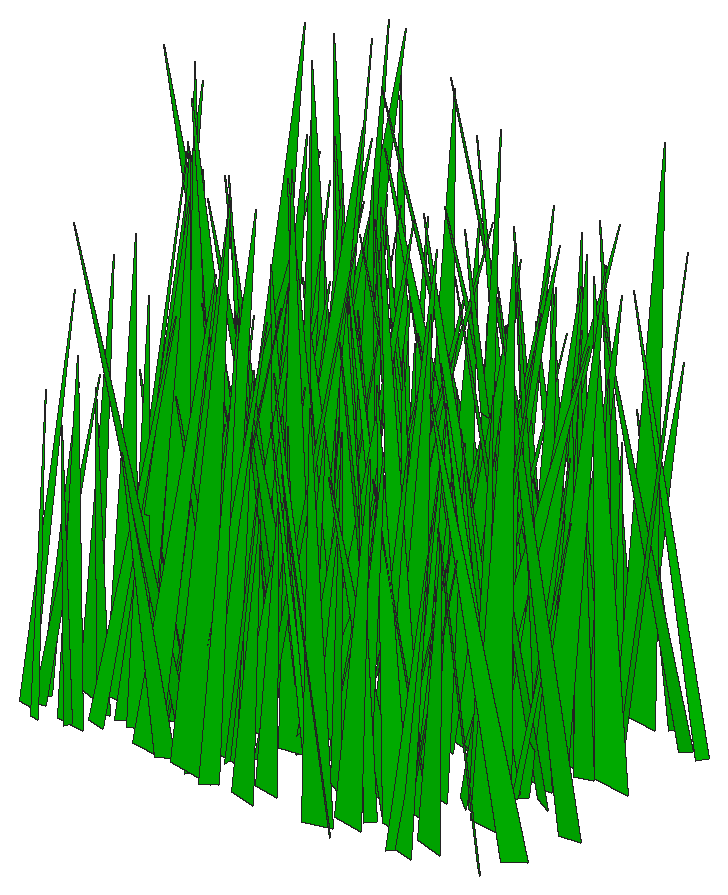
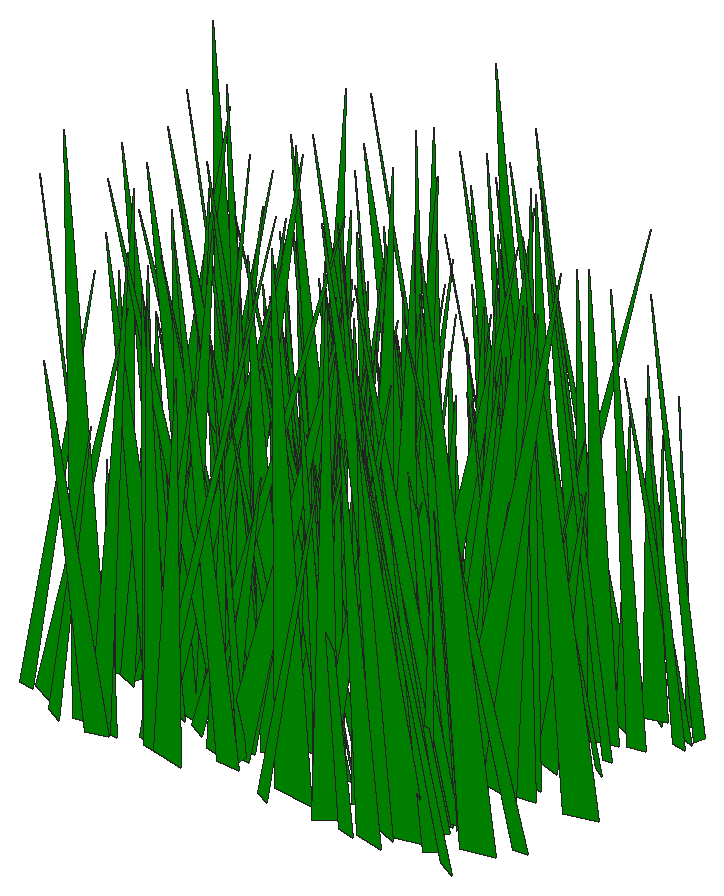
# SketchUp Ruby script. Lengths in inches.
U = 1.inch
M = Sketchup.active_model
def pt(a) = Geom::Point3d.new(a.map { |v| v * U })
def face(e, loops, mat)
  f = e.add_face(loops[0].map { |a| pt(a) })
  loops[1..].each { |l| e.add_face(l.map { |a| pt(a) }).erase! }
  f.material = f.back_material = mat if mat
  f
end
# faces: each face lists its corners as indices into pts; further lists are holes
def faces(e, pts, list, mat = nil) = list.each { |f| face(e, (f[0].is_a?(Array) ? f : [f]).map { |l| l.map { |i| pts[i] } }, mat) }
# xy, xz, yz: faces in a plane at the given z, y or x. An outline is a flat list of corners, or four numbers for a rectangle; further outlines are holes
def ring(l) = l.size == 4 ? [[l[0], l[1]], [l[2], l[1]], [l[2], l[3]], [l[0], l[3]]] : l.each_slice(2).to_a
def flat(e, list, mat, &to3) = list.each { |f| face(e, (f[0].is_a?(Array) ? f : [f]).map { |l| ring(l).map { |u, v| to3.(u, v) } }, mat) }
def xy(e, z, list, mat = nil) = flat(e, list, mat) { |x, y| [x, y, z] }
def xz(e, y, list, mat = nil) = flat(e, list, mat) { |x, z| [x, y, z] }
def yz(e, x, list, mat = nil) = flat(e, list, mat) { |y, z| [x, y, z] }
def lines(e, pts, list) = list.each { |a, b| e.add_line(pt(pts[a]), pt(pts[b])) }
# prism: a flat outline (further loops are holes) pulled along v
def prism(e, loops, v, mat = nil)
  f = face(e, loops, mat); d = Geom::Vector3d.new(v.map { |x| x * U })
  f.pushpull(f.normal.samedirection?(d) ? d.length : -d.length)
end
def box(e, o, s, mat = nil) = prism(e, [[o, [o[0] + s[0], o[1], o[2]], [o[0] + s[0], o[1] + s[1], o[2]], [o[0], o[1] + s[1], o[2]]]], [0, 0, s[2]], mat)
def at(x, y, z, deg = 0) = Geom::Transformation.translation(pt([x, y, z])) * Geom::Transformation.rotation(ORIGIN, Z_AXIS, deg.degrees)
def axes(o, x, y, z) = Geom::Transformation.new([*x, 0, *y, 0, *z, 0, *pt(o).to_a, 1])
def part(name) = M.definitions.add(name)
# library, detail: a bought-in or finely detailed component or shape, given as its bounding box
def library(name, o, s) = part(name).tap { |d| box(d.entities, o, s) }
def detail(e, o, s) = box(e.add_group.entities, o, s)
def put(e, d, t, mat = nil) = e.add_instance(d, t).tap { |i| i.material = mat if mat }
def group(e, t, mat = nil) = e.add_group.tap { |g| g.transformation = t; g.material = mat if mat }.entities
root = M.entities
M.materials.add("[Color G06]").color = [0, 204, 0]
c1 = part("fur_instance\#9")
p = [[0.8125,0,1.79],[0.67,-0.02,1.48],[0,-0.11,0],[0,0.11,0]]
faces(c1.entities,p,[[0,1,2,3]])
put(root,c1,axes([91.95,21.32,4.28],[1.64465,0.73134,2.25033],[5.45141,-0.21076,-1.03131],[0.23572,-0.22861,8.1499]),"[Color G06]")
put(root,c1,axes([92.71,15.9,4.28],[2.99438,-0.06344,1.89199],[-0.62767,-0.4469,0.49765],[-1.18975,0.07611,4.49924]),"[Color G06]")
put(root,c1,axes([92.1,16.31,4.28],[4.0526,-0.14556,1.75837],[-1.22143,-0.57694,0.80167],[-0.99093,0.11582,6.20302]),"[Color G06]")
put(root,c1,axes([92.28,16.91,4.28],[3.05677,-0.19884,0.87659],[-1.37312,-0.43367,-0.60473],[-0.70131,-0.01757,5.0048]),"[Color G06]")
put(root,c1,axes([92.375,16.52,4.28],[2.99104,0.29547,0.37118],[2.10052,-0.4183,0.44185],[-0.37328,0.01376,5.46057]),"[Color G06]")
put(root,c1,axes([94.8,22.62,4.28],[2.21877,0.53293,5.82163],[4.74581,-0.47788,0.9851],[-2.69366,-0.40297,6.5309]),"[Color G06]")
put(root,c1,axes([93.6,16.14,4.28],[2.27486,0.22768,1.51712],[1.48655,-0.34736,1.00952],[-1.21924,0.00129,4.06149]),"[Color G06]")
put(root,c1,axes([93.07,17.67,4.28],[3.03492,0.39872,2.50768],[3.18932,-0.43774,-0.62669],[-0.9051,-0.2055,6.20035]),"[Color G06]")
put(root,c1,axes([93.63,16.2,4.28],[-1.08085,0.50633,0.55689],[3.62015,0.15563,-0.55976],[0.46648,-0.03458,5.6344]),"[Color G06]")
put(root,c1,axes([94.27,19.8125,4.28],[-0.50605,0.37921,1.58428],[2.87616,0.03927,0.97251],[-0.49659,-0.15902,4.01814]),"[Color G06]")
put(root,c1,axes([92.85,24.4,4.28],[1.81921,0.75767,2.15229],[5.62004,-0.24113,-0.85976],[0.10756,-0.21572,8.52053]),"[Color G06]")
put(root,c1,axes([94.36,21.62,4.28],[1.43029,-0.58528,3.25632],[-4.53769,-0.25922,-0.90006],[-1.33139,0.25473,6.56581]),"[Color G06]")
put(root,c1,axes([93.08,19.76,4.28],[1.51262,0.3388,0.84647],[2.49354,-0.20247,-0.64393],[0.07692,-0.09865,4.22869]),"[Color G06]")
put(root,c1,axes([92.03,23.69,4.28],[4.42501,0.36233,0.30572],[2.60635,-0.61553,-0.46422],[-0.01867,-0.0518,7.65535]),"[Color G06]")
put(root,c1,axes([94,17.08,4.28],[2.06067,0.31223,1.61538],[2.21047,-0.31969,0.79948],[-1.13822,-0.05557,4.47718]),"[Color G06]")
put(root,c1,axes([93.82,21.51,4.28],[-0.60566,-0.69279,0.93666],[-4.99182,0.0905,0.47974],[0.3968,0.08111,7.4649]),"[Color G06]")
put(root,c1,axes([93.07,19.2,4.28],[2.93871,0.17543,0.30847],[1.22542,-0.40864,0.6195],[-0.3516,0.04202,4.73731]),"[Color G06]")
put(root,c1,axes([94.08,20.89,4.28],[4.11121,-0.516,3.26399],[-3.85509,-0.6291,-0.57814],[-1.89747,0.16013,8.24663]),"[Color G06]")
put(root,c1,axes([93.92,17.93,4.28],[-1.43333,0.57089,2.63425],[4.36949,0.23095,-0.43888],[0.88024,-0.21683,6.46806]),"[Color G06]")
put(root,c1,axes([92.95,25.57,4.28],[3.76983,0.29249,0.11472],[2.07066,-0.52185,0.85143],[-0.34352,0.06427,6.39126]),"[Color G06]")
put(root,c1,axes([95.07,22.84,4.28],[-2.9575,-0.53591,0.43812],[-3.81178,0.41431,0.74025],[0.57108,-0.00997,7.20988]),"[Color G06]")
put(root,c1,axes([93.25,18.61,4.28],[5.58813,-0.10913,1.7411],[-0.71926,-0.79537,-0.57038],[-1.2051,-0.03134,8.41406]),"[Color G06]")
put(root,c1,axes([94.03,23.76,4.28],[2.93262,0.05641,1.41875],[0.59159,-0.41868,-0.81912],[-0.84545,-0.09728,4.34804]),"[Color G06]")
put(root,c1,axes([93.76,25.09,4.28],[1.35656,-0.37728,0.80661],[-2.75127,-0.17878,0.72969],[0.20459,0.09739,4.46423]),"[Color G06]")
put(root,c1,axes([94.75,24.08,4.28],[-1.97383,0.26013,0.5172],[1.76197,0.27715,-0.99228],[0.70359,0.03569,3.93588]),"[Color G06]")
put(root,c1,axes([94.69,18.97,4.28],[1.16364,-0.67512,3.34217],[-5.32923,-0.15917,0.45111],[-0.19991,0.31342,7.42835]),"[Color G06]")
put(root,c1,axes([94.53,23.07,4.28],[-0.46455,0.6645,2.60656],[4.99984,0.10165,-0.98646],[0.86674,-0.23023,7.08753]),"[Color G06]")
put(root,c1,axes([94.46,21.07,4.28],[3.42196,-0.19032,0.99506],[-1.30572,-0.48562,-0.63985],[-0.77539,-0.02219,5.46887]),"[Color G06]")
put(root,c1,axes([94.74,22.9,4.28],[0.39123,-0.56087,0.88439],[-4.04925,-0.04637,0.62342],[0.36261,0.08738,6.00752]),"[Color G06]")
put(root,c1,axes([95.92,20.8,4.28],[-1.70962,0.30842,0.79986],[2.27481,0.23405,0.49352],[0.059,-0.0873,4.14878]),"[Color G06]")
put(root,c1,axes([95.11,17.1,4.28],[3.13375,-0.39209,1.95253],[-2.87491,-0.46445,-0.40724],[-1.16087,0.0918,6.27937]),"[Color G06]")
put(root,c1,axes([94.47,23.73,4.28],[4.2554,-0.27939,1.23783],[-1.95141,-0.60445,-0.68723],[-0.94461,-0.00994,6.99603]),"[Color G06]")
put(root,c1,axes([96.55,19.83,4.28],[-2.49548,0.77239,0.426],[5.54426,0.34621,0.43851],[-0.15085,-0.05302,9.06921]),"[Color G06]")
put(root,c1,axes([94.13,16.61,4.28],[4.2348,-0.19544,1.12768],[-1.51164,-0.58747,0.98408],[-0.49864,0.1211,6.59383]),"[Color G06]")
put(root,c1,axes([97.25,16.5625,4.28],[-4.59793,-0.36372,0.46774],[-2.6267,0.63798,-0.68693],[0.044,0.0773,7.87078]),"[Color G06]")
put(root,c1,axes([94.18,24.25,4.28],[3.85342,-0.32238,0.85745],[-2.37548,-0.53133,0.89846],[-0.17576,0.11325,6.65582]),"[Color G06]")
put(root,c1,axes([96.08,20.73,4.28],[-4.52783,0.15917,2.66712],[1.40693,0.66496,0.77652],[1.58369,-0.13566,6.93557]),"[Color G06]")
put(root,c1,axes([95.37,25.71,4.28],[1.86018,0.53518,0.62372],[3.82813,-0.26406,0.52574],[-0.49945,-0.03069,6.35262]),"[Color G06]")
put(root,c1,axes([95.9,22.22,4.28],[0.58753,-0.52227,1.63752],[-3.86787,-0.09841,-0.50568],[-0.51706,0.14272,5.64348]),"[Color G06]")
put(root,c1,axes([95.6875,19.57,4.28],[-2.50721,-0.37686,1.81547],[-2.6715,0.38349,0.90351],[1.28157,0.06213,5.43509]),"[Color G06]")
put(root,c1,axes([94.43,23.67,4.28],[3.53534,0.5577,0.76514],[4.03176,-0.4901,-0.57566],[-0.04827,-0.08908,7.95719]),"[Color G06]")
put(root,c1,axes([94.59,25.02,4.28],[2.2635,0.80743,1.04085],[5.81948,-0.30588,-1.01146],[0.3822,-0.12448,9.23651]),"[Color G06]")
put(root,c1,axes([96.15,23.26,4.28],[-1.78077,0.31236,0.47134],[2.21083,0.25217,-0.53936],[0.47889,-0.00264,4.24274]),"[Color G06]")
put(root,c1,axes([96.32,23.34,4.28],[0.37297,0.80273,1.56889],[5.81494,-0.06722,0.86282],[-0.65308,-0.14005,8.57838]),"[Color G06]")
put(root,c1,axes([94.71,17.29,4.28],[4.34523,-0.58439,0.34625],[-4.14669,-0.60491,-1.04009],[-0.6491,-0.04762,8.96239]),"[Color G06]")
put(root,c1,axes([95.05,21.3,4.28],[2.09902,0.42207,1.37893],[3.16426,-0.27995,-0.91564],[0.00054,-0.15444,5.42838]),"[Color G06]")
put(root,c1,axes([96.59,16.34,4.28],[-0.45543,-0.40546,0.95129],[-2.93274,0.04578,-0.89476],[-0.5087,0.09907,4.30676]),"[Color G06]")
put(root,c1,axes([96.84,17.41,4.28],[-2.89233,-0.0914,0.36995],[-0.61413,0.40129,0.6644],[0.33727,-0.05312,4.38233]),"[Color G06]")
put(root,c1,axes([95.33,25.125,4.28],[4.87842,0.45836,2.23764],[3.29222,-0.7086,0.64133],[-1.48574,-0.06514,8.76839]),"[Color G06]")
put(root,c1,axes([95.68,18.75,4.28],[-1.11238,0.64458,2.21192],[4.75124,0.18787,-0.95173],[0.99156,-0.17708,7.04181]),"[Color G06]")
put(root,c1,axes([97.89,19.89,4.28],[-4.06494,-0.02811,0.27236],[-0.22865,0.5597,-0.98594],[0.14689,0.09321,6.00238]),"[Color G06]")
put(root,c1,axes([95.63,17.9375,4.28],[4.09226,0.49238,1.39853],[3.51284,-0.58419,0.66672],[-1.00181,-0.03715,8.05069]),"[Color G06]")
put(root,c1,axes([95.69,23.86,4.28],[5.90719,-0.15838,2.43731],[-1.02526,-0.85381,-0.82302],[-1.70244,-0.03537,8.9527]),"[Color G06]")
put(root,c1,axes([96.12,25.7,4.28],[3.19355,-0.23482,0.85311],[-1.60083,-0.45093,-0.87237],[-0.7739,-0.03625,5.32493]),"[Color G06]")
put(root,c1,axes([96.95,25.49,4.28],[3.54346,-0.40804,4.40308],[-3.76669,-0.54316,0.98885],[-1.74751,0.34336,6.79678]),"[Color G06]")
put(root,c1,axes([97.75,17.88,4.28],[-1.76497,-0.43414,0.22457],[-3.10942,0.24356,-0.49855],[-0.21666,0.04111,5.32554]),"[Color G06]")
put(root,c1,axes([97.13,23.24,4.28],[3.75132,-0.61056,3.41678],[-4.53662,-0.58422,-0.86668],[-1.95359,0.18427,8.57359]),"[Color G06]")
put(root,c1,axes([96.54,24.28,4.28],[-0.44673,-0.68146,0.96305],[-4.88803,0.07288,0.85925],[0.6357,0.0815,7.28378]),"[Color G06]")
put(root,c1,axes([96.03,21.27,4.28],[1.87379,0.52475,1.07318],[3.82757,-0.25173,-0.78863],[0.16166,-0.1222,6.2332]),"[Color G06]")
put(root,c1,axes([98.05,24.19,4.28],[-3.83242,0.27082,1.38135],[2.08696,0.53192,0.95406],[0.52013,-0.13883,6.35003]),"[Color G06]")
put(root,c1,axes([98.47,19.72,4.28],[-3.59612,-0.54162,0.50753],[-3.89888,0.49945,-0.48125],[-0.00648,0.06525,7.89645]),"[Color G06]")
put(root,c1,axes([96.56,18.17,4.28],[0.81207,0.75992,0.72789],[5.46522,-0.10943,-0.49565],[0.25764,-0.07389,8.21978]),"[Color G06]")
put(root,c1,axes([97.32,19.21,4.28],[0.75766,-0.55761,1.57953],[-4.10077,-0.12081,-0.50553],[-0.53941,0.13522,6.06178]),"[Color G06]")
put(root,c1,axes([95.97,16.37,4.28],[3.6282,-0.49221,1.51641],[-3.65759,-0.50226,0.82028],[-0.33262,0.15402,7.52081]),"[Color G06]")
put(root,c1,axes([96.2,16.72,4.28],[3.48639,0.09583,0.67061],[0.6484,-0.489,0.49755],[-0.50318,0.03386,5.28758]),"[Color G06]")
put(root,c1,axes([96.81,22.35,4.28],[4.00358,0.04241,1.86246],[0.46894,-0.57849,-0.73852],[-1.19394,-0.085,5.95526]),"[Color G06]")
put(root,c1,axes([97.37,21.48,4.28],[1.89763,0.56922,1.9269],[4.20339,-0.28499,0.42443],[-0.81028,-0.14534,6.71448]),"[Color G06]")
put(root,c1,axes([96.2,23.37,4.28],[4.81694,-0.0289,1.13678],[-0.14184,-0.67775,-0.63675],[-0.77547,-0.05555,7.17774]),"[Color G06]")
put(root,c1,axes([98.3,19.2,4.28],[-3.66356,-0.29535,0.89766],[-2.03706,0.51643,0.94899],[0.83507,-0.03598,6.25309]),"[Color G06]")
put(root,c1,axes([96.22,17.97,4.28],[4.6601,0.03494,0.83555],[0.21637,-0.65342,0.44321],[-0.57316,0.03741,6.96082]),"[Color G06]")
put(root,c1,axes([96.91,21.89,4.28],[3.11215,-0.62531,0.6525],[-4.46156,-0.43803,-0.68761],[-0.62721,0.01314,8.1289]),"[Color G06]")
put(root,c1,axes([97.22,25.13,4.28],[3.51474,-0.2617,2.18796],[-2.10302,-0.51195,0.51204],[-1.11467,0.14069,5.93293]),"[Color G06]")
put(root,c1,axes([97.04,19.875,4.28],[1.73365,0.35845,0.83397],[2.63005,-0.23779,-0.47171],[-0.04451,-0.08918,4.60991]),"[Color G06]")
put(root,c1,axes([98.89,21.6,4.28],[-2.5379,0.1495,0.36355],[1.09806,0.34882,0.64508],[0.0527,-0.06869,4.06677]),"[Color G06]")
put(root,c1,axes([98.94,25.59,4.28],[-3.18182,-0.21847,0.9028],[-1.63005,0.44521,-0.45629],[0.40309,0.07582,5.28104]),"[Color G06]")
put(root,c1,axes([98.05,20,4.28],[-4.68369,-0.32627,4.29429],[-2.96612,0.71717,-0.96689],[2.22088,0.26974,7.76503]),"[Color G06]")
put(root,c1,axes([97.18,20.6,4.28],[1.74898,0.83775,0.49469],[6.00903,-0.24076,-0.61942],[0.30617,-0.06039,9.33119]),"[Color G06]")
put(root,c1,axes([97.7,17.31,4.28],[1.02984,0.50211,1.90448],[3.81912,-0.13247,-0.60111],[0.06009,-0.18614,5.56502]),"[Color G06]")
put(root,c1,axes([98.57,21.72,4.28],[-4.09565,0.42448,3.12993],[3.39886,0.60381,0.52775],[1.44907,-0.2165,7.60854]),"[Color G06]")
put(root,c1,axes([97.36,18.84,4.28],[2.99256,-0.29017,1.13786],[-2.18836,-0.41504,0.6975],[-0.34773,0.11469,5.4028]),"[Color G06]")
put(root,c1,axes([98.5,22.02,4.28],[2.51636,-0.19004,1.81097],[-1.24024,-0.38944,-0.84508],[-1.33689,0.00359,4.19271]),"[Color G06]")
put(root,c1,axes([97.61,16.125,4.28],[0.02228,0.70307,4.68772],[5.88419,0.05605,-1.0282],[0.79646,-0.43377,7.46505]),"[Color G06]")
put(root,c1,axes([98.76,20.03,4.28],[0.93266,-0.7566,1.56566],[-5.45628,-0.14954,-1.0409],[-0.87475,0.12606,8.16201]),"[Color G06]")
put(root,c1,axes([97.98,17.15,4.28],[2.66516,0.17119,0.78651],[1.10653,-0.37471,0.99352],[-0.7481,0.05563,4.27153]),"[Color G06]")
put(root,c1,axes([98.39,23.27,4.28],[-1.41919,-0.41651,0.91922],[-2.96636,0.21049,0.726],[0.70736,0.04706,4.88877]),"[Color G06]")
put(root,c1,axes([98.33,25.08,4.28],[1.4761,0.76761,1.12378],[5.53414,-0.21272,0.45425],[-0.49057,-0.09006,8.50575]),"[Color G06]")
put(root,c1,axes([98.63,24.75,4.28],[-2.2068,-0.21807,1.04001],[-1.48492,0.32265,0.73349],[0.85133,-0.00248,3.97529]),"[Color G06]")
put(root,c1,axes([98.43,23.78,4.28],[-1.98118,0.35268,1.1502],[2.45384,0.29522,-0.9575],[0.98365,-0.02614,4.70525]),"[Color G06]")
put(root,c1,axes([99.125,20.22,4.28],[-0.49134,0.44469,1.22671],[3.26056,0.04951,0.8554],[-0.46067,-0.12387,4.74598]),"[Color G06]")
put(root,c1,axes([97.53,22.77,4.28],[3.13387,-0.13497,0.45801],[-0.99727,-0.43524,0.50819],[-0.19044,0.05804,4.87571]),"[Color G06]")
put(root,c1,axes([100.03,23.51,4.28],[-4.35536,0.09656,0.82743],[0.77067,0.60368,0.9682],[0.43831,-0.1019,6.51967]),"[Color G06]")
put(root,c1,axes([98.85,18.72,4.28],[2.64629,0.14895,2.4302],[1.51659,-0.39771,-0.88866],[-1.21857,-0.1715,4.17154]),"[Color G06]")
put(root,c1,axes([99.66,20.125,4.28],[-2.03847,0.52015,1.88665],[3.93797,0.26896,0.98599],[-0.00588,-0.19861,6.27618]),"[Color G06]")
put(root,c1,axes([98.48,19.53,4.28],[0.36446,-0.40217,1.47164],[-3.03445,-0.0351,0.57672],[0.28184,0.14214,4.30626]),"[Color G06]")
put(root,c1,axes([99.07,18.62,4.28],[1.48161,0.74655,2.37301],[5.51387,-0.23181,0.68769],[-0.88324,-0.19485,8.2737]),"[Color G06]")
put(root,c1,axes([98.32,15.97,4.28],[4.13606,-0.3473,1.80889],[-2.47609,-0.59967,-0.57962],[-1.23974,0.03902,7.19257]),"[Color G06]")
put(root,c1,axes([97.64,16.25,4.28],[4.59531,-0.3301,0.53237],[-2.31211,-0.63988,-0.99706],[-0.62024,-0.06034,7.66113]),"[Color G06]")
put(root,c1,axes([100.81,24.33,4.28],[-4.02186,0.48193,0.19408],[3.4508,0.55735,0.75217],[-0.23005,-0.06499,7.88962]),"[Color G06]")
put(root,c1,axes([99.45,21.88,4.28],[-3.73003,-0.00036,1.79175],[0.16936,0.5407,0.80006],[1.18681,-0.07829,5.5171]),"[Color G06]")
put(root,c1,axes([99.62,22.98,4.28],[2.61455,-0.40861,3.55022],[-3.28205,-0.44508,-0.48555],[-1.85935,0.21106,5.84927]),"[Color G06]")
put(root,c1,axes([98.16,22.95,4.28],[3.23565,0.08858,0.60938],[0.5611,-0.44966,0.85353],[-0.5049,0.06795,4.85376]),"[Color G06]")
put(root,c1,axes([99.49,22.45,4.28],[-3.71818,-0.37291,1.92629],[-2.69894,0.5446,0.47446],[1.23637,0.06736,6.82872]),"[Color G06]")
put(root,c1,axes([97.97,23.67,4.28],[1.89484,0.51387,0.57617],[3.68226,-0.25445,-0.98062],[0.41196,-0.08922,6.11499]),"[Color G06]")
put(root,c1,axes([99,19.77,4.28],[-0.57469,0.3872,0.37092],[2.7551,0.08428,-0.57125],[0.42555,-0.02274,4.19926]),"[Color G06]")
put(root,c1,axes([100.21,21.28,4.28],[-4.43487,0.16092,1.93047],[1.35698,0.63048,0.92616],[1.07641,-0.13183,6.78605]),"[Color G06]")
put(root,c1,axes([100.85,23.9,4.28],[-2.41203,0.35942,0.31934],[2.58193,0.33225,0.60489],[-0.15102,-0.06024,5.24117]),"[Color G06]")
put(root,c1,axes([99.44,15.93,4.28],[-0.04825,-0.45111,0.02317],[-3.19754,0.00698,0.73431],[0.4915,0.00111,4.77949]),"[Color G06]")
put(root,c1,axes([99.27,18.65,4.28],[0.5699,-0.38393,0.39747],[-2.72636,-0.07157,0.79025],[0.46714,0.05068,4.12722]),"[Color G06]")
put(root,c1,axes([100.57,17.3,4.28],[-3.40365,0.08463,1.41087],[0.7378,0.4855,0.6303],[0.84565,-0.08295,5.12866]),"[Color G06]")
put(root,c1,axes([99.7,16.58,4.28],[-0.06059,-0.41869,0.65791],[-3.01651,0.01501,0.47687],[0.33124,0.06012,4.46304]),"[Color G06]")
put(root,c1,axes([102.41,23.92,4.28],[-5.77783,-0.30153,0.16469],[-2.16513,0.8043,-0.50729],[-0.01595,0.04971,9.20639]),"[Color G06]")
put(root,c1,axes([98.01,22.7,4.28],[5.07071,0.26378,0.34059],[1.90523,-0.70285,-0.82848],[-0.01847,-0.08354,8.04618]),"[Color G06]")
put(root,c1,axes([98.4375,17.84,4.28],[5.68966,-0.09614,1.04279],[-0.63784,-0.7977,-0.67405],[-0.74516,-0.05123,8.53925]),"[Color G06]")
put(root,c1,axes([99.22,22.34,4.28],[2.67202,-0.39584,1.06861],[-2.92715,-0.36291,0.90634],[-0.03516,0.13064,5.7556]),"[Color G06]")
put(root,c1,axes([98.77,20.2,4.28],[5.19698,-0.32427,0.83159],[-2.30121,-0.72872,-0.51864],[-0.64934,-0.01275,8.49357]),"[Color G06]")
put(root,c1,axes([101.33,16.78,4.28],[-3.64074,0.32921,0.44436],[2.29786,0.5061,-1.01836],[0.61795,0.05763,6.40479]),"[Color G06]")
put(root,c1,axes([99.32,23.61,4.28],[2.94786,-0.20381,0.5567],[-1.50581,-0.4042,0.81238],[-0.08614,0.0911,4.85001]),"[Color G06]")
put(root,c1,axes([100.05,23.6,4.28],[0.28779,-0.65932,1.85026],[-4.86294,-0.02131,0.81741],[0.48953,0.17595,7.03227]),"[Color G06]")
put(root,c1,axes([101.29,24.16,4.28],[-1.05253,0.37713,0.91239],[2.76369,0.13546,0.68983],[-0.22096,-0.10217,4.28213]),"[Color G06]")
put(root,c1,axes([100.15,18.91,4.28],[1.94771,-0.2804,1.44269],[-2.22261,-0.259,0.91998],[-0.18747,0.15749,4.0816]),"[Color G06]")
put(root,c1,axes([100.24,18.77,4.28],[0.36675,0.37985,0.72745],[2.70978,-0.03543,-0.92629],[0.56051,-0.07724,4.00216]),"[Color G06]")
put(root,c1,axes([102.9,25.11,4.28],[-5.77934,-0.24182,0.81091],[-1.77438,0.80543,-0.65632],[0.39158,0.08058,8.99421]),"[Color G06]")
put(root,c1,axes([100.57,22.44,4.28],[-1.03723,-0.36571,1.48549],[-2.66824,0.17419,0.76471],[0.86396,0.09892,4.14515]),"[Color G06]")
put(root,c1,axes([100.57,24.39,4.28],[3.80207,-0.07969,1.92762],[-0.73628,-0.55311,0.61739],[-1.20328,0.08666,5.71303]),"[Color G06]")
put(root,c1,axes([101.68,18.77,4.28],[-3.99591,-0.15864,1.60701],[-1.10565,0.57702,0.40224],[1.10808,0.00368,6.19646]),"[Color G06]")
put(root,c1,axes([101.83,20.95,4.28],[-3.437,0.28494,1.87877],[2.29424,0.47993,1.01368],[0.70153,-0.1735,5.88954]),"[Color G06]")
put(root,c1,axes([101.02,22.2,4.28],[2.44796,0.29452,1.38655],[2.08762,-0.36309,0.62702],[-0.9816,-0.03771,4.79139]),"[Color G06]")
put(root,c1,axes([101.01,17.77,4.28],[-2.78855,-0.25123,2.11196],[-1.80018,0.43244,0.59986],[1.41493,0.05506,4.92546]),"[Color G06]")
put(root,c1,axes([101.28,24.54,4.28],[1.60422,-0.36688,0.90151],[-2.58975,-0.23678,-0.7755],[-0.76096,0.03241,4.53975]),"[Color G06]")
put(root,c1,axes([100.27,22.03,4.28],[2.11814,-0.35676,0.27225],[-2.55065,-0.28951,0.74614],[0.27028,0.06381,4.9078]),"[Color G06]")
put(root,c1,axes([101.78,19.29,4.28],[1.43867,0.36329,1.01685],[2.52108,-0.21952,1.0419],[-0.94574,-0.03254,4.32425]),"[Color G06]")
put(root,c1,axes([102.26,15.9375,4.28],[-3.42771,-0.09529,1.00947],[-0.55558,0.48127,1.0049],[0.7839,-0.07558,5.12621]),"[Color G06]")
put(root,c1,axes([101.65,19.92,4.28],[2.77164,-0.40639,1.85195],[-2.89668,-0.41814,-0.85672],[-1.27985,0.06629,5.94959]),"[Color G06]")
put(root,c1,axes([100.65,24.84,4.28],[4.30318,-0.39722,1.03958],[-2.81675,-0.60784,-0.63548],[-0.81486,0.00347,7.68665]),"[Color G06]")
put(root,c1,axes([101.32,18.4,4.28],[3.74901,-0.01047,1.87537],[0.07835,-0.54738,-0.70107],[-1.25459,-0.06548,5.56027]),"[Color G06]")
put(root,c1,axes([102.08,25.54,4.28],[0.53987,0.57931,0.50841],[4.12625,-0.08105,0.82162],[-0.5904,-0.03672,6.20708]),"[Color G06]")
put(root,c1,axes([100.95,22.8125,4.28],[4.09954,-0.01951,1.35761],[0.01119,-0.57792,-1.02949],[-0.919,-0.09406,6.04358]),"[Color G06]")
put(root,c1,axes([101.78,16.05,4.28],[1.05403,-0.62649,0.08558],[-4.47618,-0.14713,-0.57738],[-0.38917,-0.00456,6.87278]),"[Color G06]")
put(root,c1,axes([103.81,23.48,4.28],[-4.35322,-0.40246,0.37628],[-2.89573,0.60251,-0.8041],[-0.08892,0.0819,7.76472]),"[Color G06]")
put(root,c1,axes([101.89,22.47,4.28],[-1.70723,0.49139,1.98205],[3.66449,0.2635,-0.45379],[0.86496,-0.14643,5.83465]),"[Color G06]")
put(root,c1,axes([101.62,19.09,4.28],[2.71976,0.7023,0.27363],[5.00242,-0.37973,0.892],[-0.61193,0.01722,8.50805]),"[Color G06]")
put(root,c1,axes([103.14,17.41,4.28],[-1.15604,-0.45466,0.41842],[-3.22955,0.15182,-0.98011],[-0.52824,0.06679,5.0765]),"[Color G06]")
put(root,c1,axes([101.66,19.68,4.28],[3.04674,0.22109,0.81038],[1.50149,-0.42987,0.86232],[-0.74379,0.03785,5.06028]),"[Color G06]")
put(root,c1,axes([102.78,18.44,4.28],[3.26634,-0.476,5.08849],[-4.34222,-0.53964,0.42711],[-2.095,0.37635,7.04825]),"[Color G06]")
put(root,c1,axes([103.09,23.03,4.28],[-5.34813,0.2136,2.41468],[1.67015,0.77255,0.41223],[1.47218,-0.10046,8.30436]),"[Color G06]")
put(root,c1,axes([102.86,25.1875,4.28],[-0.5015,-0.50341,1.2561],[-3.68334,0.05445,-0.77818],[-0.4148,0.12514,5.39148]),"[Color G06]")
put(root,c1,axes([103.16,23.4375,4.28],[-0.78154,-0.48769,0.04301],[-3.4473,0.10672,-0.9132],[-0.59014,0.02244,5.27751]),"[Color G06]")
put(root,c1,axes([101.96,22.15,4.28],[-4.08873,-0.50227,4.1822],[-3.90084,0.65664,0.54028],[2.36372,0.21484,8.12594]),"[Color G06]")
put(root,c1,axes([101.89,18.1875,4.28],[2.1114,0.38285,1.62936],[2.93418,-0.29344,-0.57263],[-0.34211,-0.15391,5.14472]),"[Color G06]")
put(root,c1,axes([101.84,19.04,4.28],[4.08903,-0.12303,1.94108],[-1.08281,-0.58683,0.82238],[-1.13698,0.1164,6.19767]),"[Color G06]")
put(root,c1,axes([102.04,17.32,4.28],[1.01411,-0.4756,1.58302],[-3.57039,-0.13149,0.57111],[0.08203,0.1566,5.28728]),"[Color G06]")
put(root,c1,axes([103.29,22.4,4.28],[-3.89679,-0.48029,1.0827],[-3.39477,0.55268,0.87128],[0.92917,0.00498,7.72394]),"[Color G06]")
put(root,c1,axes([102.5,25.44,4.28],[2.04432,0.55439,1.69919],[4.04715,-0.30453,0.53746],[-0.8482,-0.11687,6.65987]),"[Color G06]")
put(root,c1,axes([102.74,16.99,4.28],[-2.79719,0.19062,2.18267],[1.66088,0.41643,0.57682],[1.11481,-0.14213,4.61721]),"[Color G06]")
put(root,c1,axes([102.36,16.56,4.28],[0.37862,-0.51111,1.44085],[-3.7774,-0.03991,0.59089],[0.30801,0.1388,5.47538]),"[Color G06]")
put(root,c1,axes([101.66,21.25,4.28],[3.69536,0.49897,1.55488],[3.71418,-0.50973,-0.92713],[-0.30167,-0.16358,7.63179]),"[Color G06]")
put(root,c1,axes([103.35,23.39,4.28],[-2.73951,-0.6019,1.21268],[-4.31567,0.39367,0.66814],[0.81529,0.06134,7.61154]),"[Color G06]")
put(root,c1,axes([104.42,20.32,4.28],[-3.57748,0.60307,0.89745],[4.36611,0.49501,0.66591],[0.03625,-0.10414,8.36208]),"[Color G06]")
put(root,c1,axes([103.51,17.07,4.28],[-2.61642,0.52014,0.36544],[3.68497,0.36588,-0.8909],[0.62791,0.02013,6.75107]),"[Color G06]")
put(root,c1,axes([102.54,18.73,4.28],[0.5412,-0.66744,1.87095],[-4.93882,-0.06254,0.62837],[0.29154,0.1796,7.17177]),"[Color G06]")
put(root,c1,axes([102.96,24.82,4.28],[-1.56615,0.59799,1.21148],[4.28001,0.23393,-0.90515],[0.85338,-0.07581,6.76296]),"[Color G06]")
put(root,c1,axes([101.54,22.55,4.28],[4.38792,0.15689,0.56469],[1.16554,-0.60769,-0.8353],[-0.2239,-0.08874,6.7185]),"[Color G06]")
put(root,c1,axes([102.12,21.51,4.28],[1.7097,0.71847,0.20895],[5.12057,-0.23442,-0.99472],[0.5882,-0.0476,8.05223]),"[Color G06]")
put(root,c1,axes([102.84,18.63,4.28],[3.7427,-0.12735,1.92339],[-1.10087,-0.54165,0.66524],[-1.13061,0.10583,5.7193]),"[Color G06]")
put(root,c1,axes([101.49,23.7,4.28],[4.36131,0.49254,0.25031],[3.53412,-0.6059,-0.58933],[0.11845,-0.05741,8.36714]),"[Color G06]")
put(root,c1,axes([104.39,17.47,4.28],[-3.42038,-0.04589,0.72051],[-0.28354,0.47993,0.50477],[0.51021,-0.04093,5.11074]),"[Color G06]")
put(root,c1,axes([101.73,21.9,4.28],[3.60302,-0.62278,0.47575],[-4.46608,-0.49583,0.99157],[0.31862,0.09249,8.51876]),"[Color G06]")
put(root,c1,axes([103.25,21.58,4.28],[-1.09257,0.39978,1.44473],[2.9182,0.17708,-0.69943],[0.7987,-0.10012,4.53181]),"[Color G06]")
put(root,c1,axes([103.17,19.05,4.28],[0.22653,0.49833,1.15609],[3.63894,-0.02017,-0.59393],[0.35711,-0.11057,5.31876]),"[Color G06]")
put(root,c1,axes([103.34,23.54,4.28],[3.168,0.36659,1.12223],[2.54523,-0.45396,0.98535],[-0.99833,0.00591,6.07331]),"[Color G06]")
put(root,c1,axes([102.83,17.72,4.28],[2.95295,0.0388,0.43446],[0.32722,-0.40627,-0.80005],[-0.2342,-0.07841,4.36016]),"[Color G06]")
put(root,c1,axes([104.32,20.17,4.28],[-2.92689,-0.29194,0.96436],[-2.04946,0.41793,0.63984],[0.77411,0.00265,5.34018]),"[Color G06]")
put(root,c1,axes([104.3,25.5,4.28],[-3.37021,-0.46933,1.79073],[-3.39005,0.4926,0.57909],[1.12731,0.07825,7.09503]),"[Color G06]")
put(root,c1,axes([104.02,25.4375,4.28],[2.04001,-0.22654,1.20551],[-1.62507,-0.30346,-0.40806],[-0.80553,0.03851,3.87617]),"[Color G06]")
put(root,c1,axes([103.68,17.94,4.28],[1.96291,-0.35689,2.21218],[-2.93098,-0.2674,0.85363],[-0.3879,0.21452,4.74443]),"[Color G06]")
put(root,c1,axes([103.77,22.34,4.28],[-0.02185,0.60026,2.88863],[4.70047,0.02638,-0.55018],[0.41329,-0.26824,6.41008]),"[Color G06]")
put(root,c1,axes([105.24,22.79,4.28],[-2.809,0.10085,0.09434],[0.71061,0.38916,-0.52651],[0.14853,0.04541,4.30309]),"[Color G06]")
put(root,c1,axes([105.6,20.43,4.28],[-4.78377,-0.28171,0.86283],[-1.9861,0.67162,0.59322],[0.68564,-0.02007,7.73842]),"[Color G06]")
put(root,c1,axes([102.625,21.4,4.28],[3.32425,0.49147,0.13692],[3.49907,-0.45775,-1.01584],[0.4323,-0.07424,7.16938]),"[Color G06]")
put(root,c1,axes([105.51,18.81,4.28],[-3.75314,0.37365,0.36468],[2.65034,0.52347,-0.68382],[0.46383,0.03233,6.85822]),"[Color G06]")
put(root,c1,axes([104.06,21.99,4.28],[0.1667,0.38235,0.07779],[2.71889,-0.02209,-0.5416],[0.35864,-0.01025,4.06972]),"[Color G06]")
put(root,c1,axes([103.61,23.89,4.28],[2.7635,-0.52121,1.18425],[-3.81742,-0.3824,0.56463],[-0.16135,0.12032,6.92443]),"[Color G06]")
put(root,c1,axes([105.16,21.03,4.28],[3.48557,0.34154,3.42547],[2.63882,-0.56374,0.45907],[-2.07091,-0.14348,6.35043]),"[Color G06]")
put(root,c1,axes([104.09,16.2,4.28],[2.81319,-0.21429,0.71109],[-1.50875,-0.39783,-0.43938],[-0.55827,-0.0047,4.77076]),"[Color G06]")
put(root,c1,axes([103.98,16.8125,4.28],[3.05215,0.0598,0.65281],[0.32701,-0.42113,1.01656],[-0.51746,0.0866,4.49291]),"[Color G06]")
put(root,c1,axes([104.54,22.47,4.28],[-0.11407,-0.50068,1.27791],[-3.67429,0.0267,0.46918],[0.34957,0.11729,5.3484]),"[Color G06]")
put(root,c1,axes([104.45,16.1875,4.28],[1.41507,0.30532,1.33696],[2.3534,-0.19627,-0.41512],[-0.23616,-0.12639,3.87419]),"[Color G06]")
put(root,c1,axes([104.08,21.3,4.28],[1.4709,0.71338,0.36206],[5.11503,-0.20284,-0.50663],[0.25931,-0.04547,7.93965]),"[Color G06]")
put(root,c1,axes([104.6875,18.94,4.28],[2.82887,0.36781,2.72273],[3.05713,-0.41147,-0.70966],[-0.9644,-0.22546,5.73699]),"[Color G06]")
put(root,c1,axes([105.43,22.99,4.28],[-2.23803,-0.26922,1.83562],[-2.21381,0.31535,-0.71609],[0.57876,0.16517,4.35911]),"[Color G06]")
put(root,c1,axes([104.29,25.64,4.28],[1.07645,0.50442,0.60655],[3.62342,-0.14286,-0.71605],[0.34703,-0.07297,5.59499]),"[Color G06]")
put(root,c1,axes([104.73,16.89,4.28],[-0.7318,-0.4648,0.31439],[-3.2633,0.1059,1.01827],[0.71092,0.00766,4.9977]),"[Color G06]")
put(root,c1,axes([104.73,25.28,4.28],[0.95098,0.7524,3.03853],[5.76579,-0.12187,-0.56428],[0.04455,-0.28828,8.16903]),"[Color G06]")
put(root,c1,axes([105.79,25.52,4.28],[-2.4432,-0.23163,1.36916],[-1.85207,0.33631,-0.84647],[0.41014,0.13887,4.33366]),"[Color G06]")
put(root,c1,axes([103.96,19.24,4.28],[5.13002,0.15036,1.57403],[1.22613,-0.71929,-1.03326],[-0.87659,-0.12617,7.76629]),"[Color G06]")
put(root,c1,axes([106.7,24.84,4.28],[-3.63629,-0.33093,0.87855],[-2.44237,0.49838,-1.01548],[0.11147,0.12431,6.40979]),"[Color G06]")
put(root,c1,axes([106.87,17.67,4.28],[-2.66838,0.52542,0.24649],[3.74459,0.36572,0.99658],[-0.45019,-0.07234,6.82826]),"[Color G06]")
put(root,c1,axes([105.57,22.13,4.28],[2.15341,0.4481,1.96646],[3.28288,-0.33307,0.68839],[-1.13139,-0.11356,5.74025]),"[Color G06]")
put(root,c1,axes([104.86,21.69,4.28],[2.72323,0.67036,0.46217],[4.79322,-0.38201,0.56334],[-0.48054,-0.01148,8.23836]),"[Color G06]")
put(root,c1,axes([105,20.39,4.28],[3.06143,0.27954,0.64466],[1.93164,-0.42942,0.89999],[-0.68809,0.03824,5.39465]),"[Color G06]")
put(root,c1,axes([105.36,18.6,4.28],[-0.82695,0.75099,3.27744],[5.76273,0.14712,-0.62459],[0.7771,-0.29182,8.11944]),"[Color G06]")
put(root,c1,axes([105.5625,22.75,4.28],[-0.64897,-0.53145,1.57542],[-3.91378,0.10759,0.5681],[0.56448,0.13498,5.7501]),"[Color G06]")
put(root,c1,axes([106.46,16.75,4.28],[-3.2136,-0.1235,1.02058],[-0.78087,0.4552,0.8352],[0.80055,-0.05174,4.91151]),"[Color G06]")
put(root,c1,axes([104.88,20.15,4.28],[3.18456,-0.10594,0.27582],[-0.71689,-0.43875,-0.87027],[-0.31199,-0.07323,4.81512]),"[Color G06]")
put(root,c1,axes([106.39,22.2,4.28],[-2.51388,0.64197,0.3798],[4.5728,0.3523,-0.79848],[0.59061,0.00481,7.79888]),"[Color G06]")
put(root,c1,axes([107.25,19.46,4.28],[-3.93306,-0.48677,1.57857],[-3.60701,0.55119,-0.54969],[0.53899,0.13665,7.84034]),"[Color G06]")
put(root,c1,axes([105.1875,24.18,4.28],[4.9125,0.19333,1.55734],[1.30768,-0.6996,0.76256],[-1.13924,0.03062,7.59068]),"[Color G06]")
put(root,c1,axes([107.29,24.77,4.28],[-4.22481,0.19079,1.29002],[1.4667,0.59376,0.6418],[0.68252,-0.09494,6.60605]),"[Color G06]")
